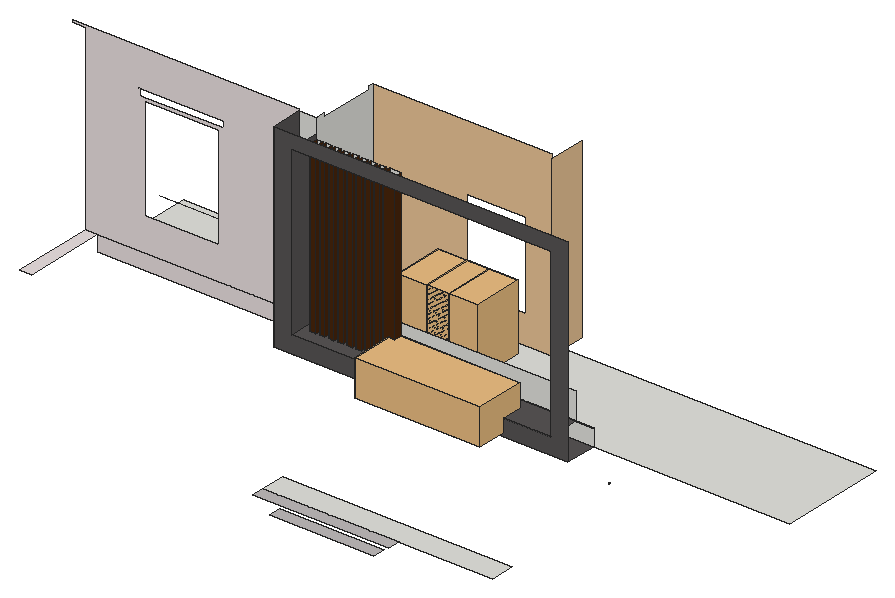
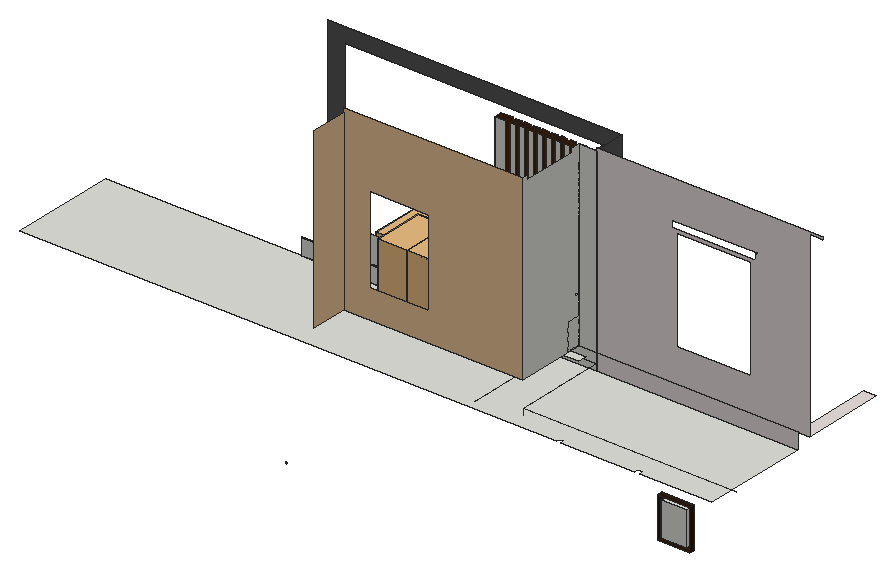
# SketchUp Ruby script. Lengths in inches.
U = 1.inch
M = Sketchup.active_model
def pt(a) = Geom::Point3d.new(a.map { |v| v * U })
def face(e, loops, mat)
  f = e.add_face(loops[0].map { |a| pt(a) })
  loops[1..].each { |l| e.add_face(l.map { |a| pt(a) }).erase! }
  f.material = f.back_material = mat if mat
  f
end
# faces: each face lists its corners as indices into pts; further lists are holes
def faces(e, pts, list, mat = nil) = list.each { |f| face(e, (f[0].is_a?(Array) ? f : [f]).map { |l| l.map { |i| pts[i] } }, mat) }
# xy, xz, yz: faces in a plane at the given z, y or x. An outline is a flat list of corners, or four numbers for a rectangle; further outlines are holes
def ring(l) = l.size == 4 ? [[l[0], l[1]], [l[2], l[1]], [l[2], l[3]], [l[0], l[3]]] : l.each_slice(2).to_a
def flat(e, list, mat, &to3) = list.each { |f| face(e, (f[0].is_a?(Array) ? f : [f]).map { |l| ring(l).map { |u, v| to3.(u, v) } }, mat) }
def xy(e, z, list, mat = nil) = flat(e, list, mat) { |x, y| [x, y, z] }
def xz(e, y, list, mat = nil) = flat(e, list, mat) { |x, z| [x, y, z] }
def yz(e, x, list, mat = nil) = flat(e, list, mat) { |y, z| [x, y, z] }
def lines(e, pts, list) = list.each { |a, b| e.add_line(pt(pts[a]), pt(pts[b])) }
# prism: a flat outline (further loops are holes) pulled along v
def prism(e, loops, v, mat = nil)
  f = face(e, loops, mat); d = Geom::Vector3d.new(v.map { |x| x * U })
  f.pushpull(f.normal.samedirection?(d) ? d.length : -d.length)
end
def box(e, o, s, mat = nil) = prism(e, [[o, [o[0] + s[0], o[1], o[2]], [o[0] + s[0], o[1] + s[1], o[2]], [o[0], o[1] + s[1], o[2]]]], [0, 0, s[2]], mat)
def at(x, y, z, deg = 0) = Geom::Transformation.translation(pt([x, y, z])) * Geom::Transformation.rotation(ORIGIN, Z_AXIS, deg.degrees)
def axes(o, x, y, z) = Geom::Transformation.new([*x, 0, *y, 0, *z, 0, *pt(o).to_a, 1])
def part(name) = M.definitions.add(name)
# library, detail: a bought-in or finely detailed component or shape, given as its bounding box
def library(name, o, s) = part(name).tap { |d| box(d.entities, o, s) }
def detail(e, o, s) = box(e.add_group.entities, o, s)
def put(e, d, t, mat = nil) = e.add_instance(d, t).tap { |i| i.material = mat if mat }
def group(e, t, mat = nil) = e.add_group.tap { |g| g.transformation = t; g.material = mat if mat }.entities
root = M.entities
M.materials.add("Generic\#1").color = [72, 38, 12]
M.materials.add("Generic\#2").color = [87, 84, 84]
M.materials.add("Generic\#3").color = [43, 24, 10]
M.materials.add("Generic\#5").color = [191, 186, 186]
M.materials.add("Generic\#8").color = [235, 197, 151]
M.materials.add("Generic\#9").color = [233, 223, 223]
M.materials.add("Material \#1").color = [140, 140, 140]
M.materials.add("[Translucent Glass Blue]").color = [100, 149, 237]
M.materials["[Translucent Glass Blue]"].alpha = 0.5
c1 = library("Plant+2 (1)",[-9.13,-9.52,0],[51.76,51.77,66.88])
c2 = library("Plante \#58",[-0.43,-1.58,0],[20.84,18.06,17.59])
xy(root,48.5625,[[238.79,67.75,304.54,75.375]],"Generic\#5")
xy(root,56.4375,[[228.29,75.375,372.83,90.9375]])
xy(root,56.4375,[[228.29,67.75,313.79,75.375]],"Generic\#5")
xy(root,82.4,[[96.84,191.625,117.22,194.8125]],"Generic\#3")
xy(root,84.54,[[98.99,191.625,115.07,194.8125]])
xy(root,105.87,[[98.99,191.625,115.07,194.8125]])
xy(root,108.02,[[96.84,191.625,117.22,194.8125]],"Generic\#3")
xy(root,115.8125,[[82.8125,127.4375,82.8125,194.8125,128.625,194.8125,128.625,192.5,131.625,192.5,131.625,194.8125,177.9375,194.8125,177.9375,192.5,180.9375,192.5,180.9375,194.8125,518.6875,194.8125,518.6875,127.4375]])
xy(root,115.8125,[[209.66,107.5625,394.85,127.4375]],"Generic\#2")
xy(root,121.625,[[216.36,121.11,228.29,133.18]])
xy(root,126,[[75.375,75.375,82.8125,127.4375]],"Generic\#9")
xy(root,126.47,[[[220.54,107.5625,383.85,127.4375],[271.44,116.13,278.63,121.07],[225.63,116.13,229.38,121.07],[231.32,116.13,235.07,121.07],[237,116.13,240.75,121.07],[242.69,116.13,246.44,121.07],[248.38,116.13,252.13,121.07],[254.07,116.13,257.82,121.07],[265.44,116.13,269.19,121.07],[259.75,116.13,263.5,121.07]]],"Generic\#2")
xz(root,107.5625,[[[209.66,115.8125,394.85,240],[220.54,126.47,383.85,231]]],"Generic\#2")
xz(root,116.13,[[225.63,126.47,229.38,232.22],[231.32,126.47,235.07,232.22],[237,126.47,240.75,232.22],[242.69,126.47,246.44,232.22],[248.38,126.47,252.13,232.22],
  [254.07,126.47,257.82,232.22],[259.75,126.47,263.5,232.22],[265.44,126.47,269.19,232.22],[271.44,126.47,278.63,232.22]],"Generic\#1")
xz(root,121.07,[[225.63,126.47,229.38,232.22],[231.32,126.47,235.07,232.22],[237,126.47,240.75,232.22],[242.69,126.47,246.44,232.22],[248.38,126.47,252.13,232.22],
  [254.07,126.47,257.82,232.22],[259.75,126.47,263.5,232.22],[265.44,126.47,269.19,232.22],[271.44,126.47,278.63,232.22]])
xz(root,127.4375,[[209.66,115.8125,232.6,120],[232.6,115.8125,232.6,120,209.66,120,209.66,126,394.85,126,394.85,115.8125],[209.66,126,220.54,240],[220.54,126,394.85,126.47],[220.54,126.47,383.85,143.28]])
xz(root,127.4375,[[82.8125,115.8125,209.66,126],[[75.375,126,209.66,126,209.66,241.3125,67.11,241.3125,67.11,240,75.375,240],[112.41,146.92,158.88,211.52],[110.52,213.3,110.38,213.31,110.23,213.33,110.1,213.38,109.96,213.44,109.84,213.52,109.73,213.61,109.63,213.72,109.54,213.84,109.47,213.97,109.42,214.1,109.38,214.25,109.37,214.39,109.22,216.98,108.1,216.92,108.02,218.23,109.15,218.29,109.16,217.98,162.04,217.98,162.02,218.29,162.71,218.33,162.78,217.02,162.1,216.98,162.25,214.24,162.25,214.125,162.23,214,162.2,213.89,162.15,213.78,162.08,213.67,162.01,213.58,161.92,213.5,161.82,213.43,161.71,213.37,161.59,213.33,161.48,213.31,161.35,213.3]]],"Generic\#9")
xz(root,171.4375,[[[220.54,126,333.65,240],[279.74,144.25,317.36,198.6875]]],"Generic\#8")
xz(root,191.625,[[[96.84,82.4,117.22,108.02],[98.99,84.54,115.07,105.87]]],"Generic\#3")
xz(root,191.625,[[98.99,84.54,115.07,105.87]],"[Translucent Glass Blue]")
xz(root,194.8125,[[98.99,84.54,115.07,105.87]])
xz(root,199.31,[[347.1,46.74,347.11,46.88,347.11,46.74],[347.74,46.82,347.7,46.83,347.71,46.84],[347.7,46.83,347.67,46.85,347.71,46.84],[347.71,46.84,347.67,46.85,347.68,46.86],[347.67,46.85,347.64,46.88,347.68,46.86],
  [347.68,46.86,347.64,46.88,347.65,46.89],[347.64,46.88,347.62,46.92,347.65,46.89],[347.65,46.89,347.62,46.92,347.625,46.92],[347.62,46.92,347.6,46.95,347.625,46.92],[347.625,46.92,347.6,46.95,347.61,46.96],
  [347.6,46.95,347.59,47,347.61,46.96],[347.61,46.96,347.59,47,347.6,47],[347.16,47,347.2,47.12,347.21,47.11],[347.59,47,347.58,47.05,347.6,47],[347.6,47,347.58,47.05,347.6,47.05],
  [347.58,47.05,347.59,47.09,347.6,47.05],[347.6,47.05,347.59,47.09,347.6,47.08],[347.6,47.08,347.59,47.09,347.6,47.13],[347.6,47.08,347.6,47.13,347.61,47.12],[347.21,47.11,347.2,47.12,347.27,47.23],
  [347.21,47.11,347.27,47.23,347.28,47.22],[347.61,47.12,347.6,47.13,347.62,47.17],[347.61,47.12,347.62,47.17,347.625,47.16],[347.625,47.16,347.62,47.17,347.64,47.2],[347.28,47.22,347.27,47.23,347.36,47.3125],
  [347.78,47.27,347.78,47.28,347.82,47.29],[347.78,47.27,347.82,47.29,347.82,47.28],[347.36,47.3,347.46,47.39,347.46,47.375],[347.7,47.46,347.69,47.47,347.82,47.49],[347.7,47.46,347.82,47.49,347.82,47.47]],"Material \#1")
yz(root,96.84,[[191.625,82.4,194.8125,108.02]],"Generic\#3")
yz(root,98.99,[[191.625,84.54,194.8125,105.87]])
yz(root,115.07,[[191.625,84.54,194.8125,105.87]])
yz(root,117.22,[[191.625,82.4,194.8125,108.02]],"Generic\#3")
yz(root,209.66,[[107.5625,115.8125,127.4375,240]],"Generic\#2")
yz(root,220.54,[[[127.4375,126,171.4375,126,171.4375,240,168.26,240,168.26,237.6875,133.36,237.6875,133.36,240,127.4375,240,127.4375,143.28,136.1875,143.28,136.1875,126.47,127.4375,126.47],[128.02,155.04,130.65,156.97],[131.35,150.72,130.82,150.75,130.19,150.75,130.19,151.1875,130.82,151.1875,130.82,151.0625,130.82,151.1875,131.36,151.16,131.35,151.04],[131.35,148.72,130.82,148.75,130.19,148.75,130.19,149.1875,130.82,149.1875,130.82,149.0625,130.82,149.1875,131.36,149.16,131.35,149.04],[131.35,152.72,130.82,152.75,130.19,152.75,130.19,153.1875,130.82,153.1875,130.82,153.0625,130.82,153.1875,131.36,153.16,131.35,153.04]],[127.4375,126.47,136.1875,143.28]])
yz(root,220.54,[[107.5625,126.47,127.4375,231]],"Generic\#2")
yz(root,225.63,[[116.13,126.47,121.07,232.22]],"Generic\#1")
yz(root,229.38,[[116.13,126.47,121.07,232.22]],"Generic\#1")
yz(root,231.32,[[116.13,126.47,121.07,232.22]],"Generic\#1")
yz(root,235.07,[[116.13,126.47,121.07,232.22]],"Generic\#1")
yz(root,237,[[116.13,126.47,121.07,232.22]],"Generic\#1")
yz(root,240.75,[[116.13,126.47,121.07,232.22]],"Generic\#1")
yz(root,242.69,[[116.13,126.47,121.07,232.22]],"Generic\#1")
yz(root,246.44,[[116.13,126.47,121.07,232.22]],"Generic\#1")
yz(root,248.38,[[116.13,126.47,121.07,232.22]],"Generic\#1")
yz(root,252.13,[[116.13,126.47,121.07,232.22]],"Generic\#1")
yz(root,254.07,[[116.13,126.47,121.07,232.22]],"Generic\#1")
yz(root,257.82,[[116.13,126.47,121.07,232.22]],"Generic\#1")
yz(root,259.75,[[116.13,126.47,121.07,232.22]],"Generic\#1")
yz(root,263.5,[[116.13,126.47,121.07,232.22]],"Generic\#1")
yz(root,265.44,[[116.13,126.47,121.07,232.22]],"Generic\#1")
yz(root,269.19,[[116.13,126.47,121.07,232.22]],"Generic\#1")
yz(root,271.44,[[116.13,126.47,121.07,232.22]],"Generic\#1")
yz(root,278.63,[[116.13,126.47,121.07,232.22]],"Generic\#1")
yz(root,333.65,[[171.4375,126,194.75,237.1875]],"Generic\#8")
p = [[232.6,127.4375,120],[232.6,194.8125,120],[209.66,127.4375,120],[209.66,184.9375,120],[75.375,184.9375,120],[209.66,184.9375,115.8125]]
lines(root,p,[[0,1],[2,3],[4,3],[3,5]])
put(root,c1,axes([274.29,136.95,126],[0.6188,0,0],[0,0.6188,0],[0,0,0.6188]))
put(root,c1,axes([292.54,136.95,126],[0.6188,0,0],[0,0.6188,0],[0,0,0.6188]))
put(root,c2,axes([276.59,92.25,117.94],[3.7878,0,0],[0,1.74,0],[0,0,1.28]))
